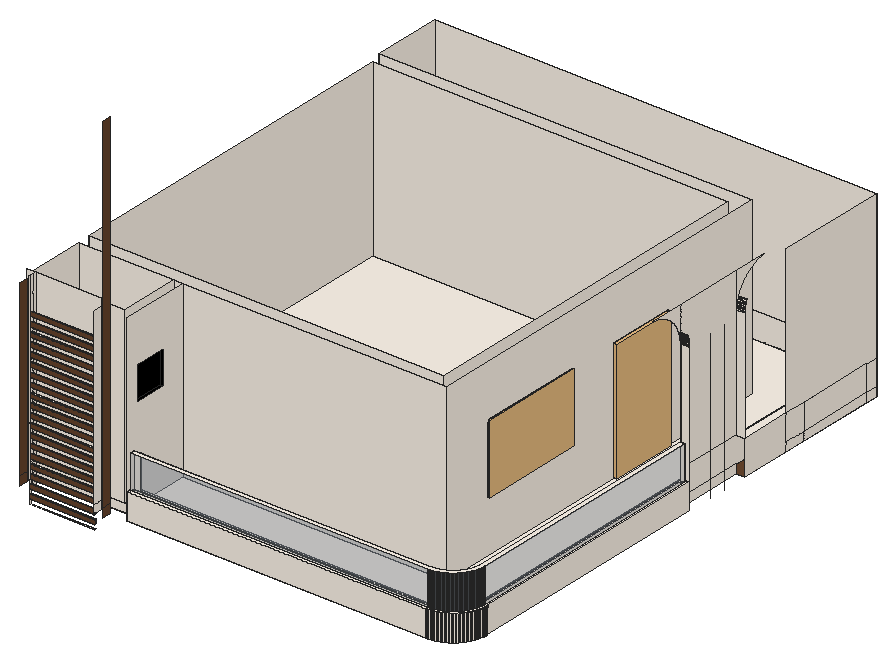
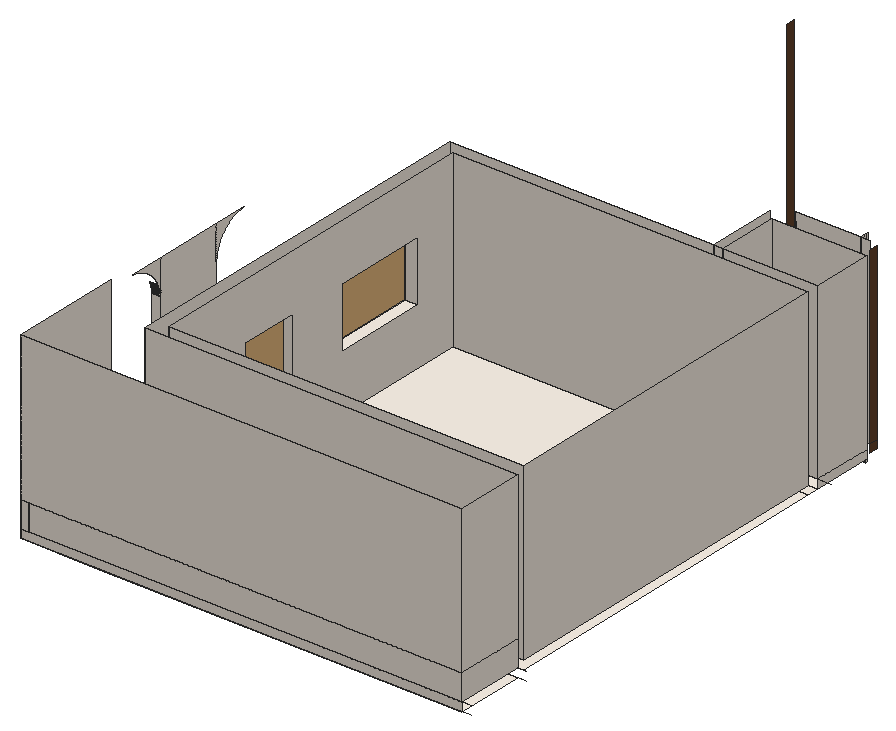
# SketchUp Ruby script. Lengths in inches.
U = 1.inch
M = Sketchup.active_model
def pt(a) = Geom::Point3d.new(a.map { |v| v * U })
def face(e, loops, mat)
  f = e.add_face(loops[0].map { |a| pt(a) })
  loops[1..].each { |l| e.add_face(l.map { |a| pt(a) }).erase! }
  f.material = f.back_material = mat if mat
  f
end
# faces: each face lists its corners as indices into pts; further lists are holes
def faces(e, pts, list, mat = nil) = list.each { |f| face(e, (f[0].is_a?(Array) ? f : [f]).map { |l| l.map { |i| pts[i] } }, mat) }
# xy, xz, yz: faces in a plane at the given z, y or x. An outline is a flat list of corners, or four numbers for a rectangle; further outlines are holes
def ring(l) = l.size == 4 ? [[l[0], l[1]], [l[2], l[1]], [l[2], l[3]], [l[0], l[3]]] : l.each_slice(2).to_a
def flat(e, list, mat, &to3) = list.each { |f| face(e, (f[0].is_a?(Array) ? f : [f]).map { |l| ring(l).map { |u, v| to3.(u, v) } }, mat) }
def xy(e, z, list, mat = nil) = flat(e, list, mat) { |x, y| [x, y, z] }
def xz(e, y, list, mat = nil) = flat(e, list, mat) { |x, z| [x, y, z] }
def yz(e, x, list, mat = nil) = flat(e, list, mat) { |y, z| [x, y, z] }
def lines(e, pts, list) = list.each { |a, b| e.add_line(pt(pts[a]), pt(pts[b])) }
# prism: a flat outline (further loops are holes) pulled along v
def prism(e, loops, v, mat = nil)
  f = face(e, loops, mat); d = Geom::Vector3d.new(v.map { |x| x * U })
  f.pushpull(f.normal.samedirection?(d) ? d.length : -d.length)
end
def box(e, o, s, mat = nil) = prism(e, [[o, [o[0] + s[0], o[1], o[2]], [o[0] + s[0], o[1] + s[1], o[2]], [o[0], o[1] + s[1], o[2]]]], [0, 0, s[2]], mat)
def at(x, y, z, deg = 0) = Geom::Transformation.translation(pt([x, y, z])) * Geom::Transformation.rotation(ORIGIN, Z_AXIS, deg.degrees)
def axes(o, x, y, z) = Geom::Transformation.new([*x, 0, *y, 0, *z, 0, *pt(o).to_a, 1])
def part(name) = M.definitions.add(name)
# library, detail: a bought-in or finely detailed component or shape, given as its bounding box
def library(name, o, s) = part(name).tap { |d| box(d.entities, o, s) }
def detail(e, o, s) = box(e.add_group.entities, o, s)
def put(e, d, t, mat = nil) = e.add_instance(d, t).tap { |i| i.material = mat if mat }
def group(e, t, mat = nil) = e.add_group.tap { |g| g.transformation = t; g.material = mat if mat }.entities
root = M.entities
M.materials.add("C01_Vanilla_Cream").color = [255, 246, 235]
M.materials.add("Glass_Basic_01").color = [161, 173, 186]
M.materials["Glass_Basic_01"].alpha = 0.25
M.materials.add("Wood_Veneer_15_1K").color = [103, 69, 45]
M.materials.add("[Color_009]1").color = [0, 0, 0]
c1 = library("porta+4",[0.2,-5.42,1.33],[46.55,4.72,83.21])
c2 = library("mesh-164",[-1582.71,-3144.16,-23.22],[2366.42,2227.34,65.81])
c3 = part("Group13")
put(c3.entities,c2,at(294.66,859.51,3.5))
xy(root,386.25,[[66,1,111,2]],"C01_Vanilla_Cream")
xy(root,389.4,[[66,1,111,2]],"C01_Vanilla_Cream")
xy(root,392.55,[[66,1,111,2]],"C01_Vanilla_Cream")
xy(root,395.7,[[66,1,111,2]],"C01_Vanilla_Cream")
xy(root,396,[[57,12,123,54],[123,12,129,54],[57,54,312,63],[57,63,303,309],[303,63,312,309],
  [54,318,312,366]],"C01_Vanilla_Cream")
xy(root,396,[[129,6,129,54,312,54,312,366,360,366,360,252,354,252,354,204,360,204,360,30,359.99,29.25,359.95,28.49,359.89,27.74,359.8125,26.99,359.7,26.25,359.57,25.5,359.42,24.76,359.25,24.03,359.05,23.3,358.83,22.58,358.58,21.87,358.31,21.17,358.03,20.47,357.72,19.78,357.38,19.1,357.03,18.4375,356.66,17.78,356.26,17.14,355.85,16.51,355.42,15.89,354.96,15.29,354.49,14.7,354,14.13,353.5,13.57,352.97,13.03,352.43,12.5,351.87,12,351.3,11.51,350.71,11.04,350.11,10.58,349.49,10.15,348.86,9.74,348.22,9.34,347.5625,8.97,346.9,8.62,346.22,8.28,345.53,7.97,344.83,7.69,344.13,7.42,343.42,7.17,342.7,6.95,341.97,6.75,341.24,6.58,340.5,6.43,339.75,6.3,339.01,6.1875,338.26,6.11,337.51,6.05,336.75,6.01,336,6]],"Wood_Veneer_15_1K")
xy(root,398.85,[[66,1,111,2]],"C01_Vanilla_Cream")
xy(root,402,[[66,1,111,2],[129,12,336,12,336.57,12.01,337.13,12.04,337.69,12.08,338.26,12.14,338.82,12.22,339.37,12.32,339.93,12.43,340.48,12.57,341.02,12.71,341.5625,12.88,342.1,13.0625,342.625,13.26,343.15,13.48,343.66,13.71,344.17,13.96,344.67,14.23,345.16,14.51,345.64,14.8,346.12,15.11,346.58,15.4375,347.03,15.78,347.47,16.13,347.9,16.5,348.32,16.88,348.73,17.27,349.12,17.68,349.5,18.1,349.87,18.53,350.22,18.97,350.5625,19.42,350.89,19.88,351.2,20.36,351.49,20.84,351.77,21.33,352.04,21.83,352.29,22.34,352.52,22.85,352.74,23.375,352.9375,23.9,353.12,24.4375,353.29,24.98,353.43,25.52,353.57,26.07,353.68,26.63,353.78,27.18,353.86,27.74,353.92,28.31,353.96,28.87,353.99,29.43,354,30,354,366,54,366,54,318,312,318,312,54,129,54],[57,12,123,54],[123,12,129,54],[57,63,303,309]],"C01_Vanilla_Cream")
xy(root,405,[[303,201,312,243]],"C01_Vanilla_Cream")
xy(root,405.15,[[66,1,111,2]],"C01_Vanilla_Cream")
xy(root,408.3,[[66,1,111,2]],"C01_Vanilla_Cream")
xy(root,411.45,[[66,1,111,2]],"C01_Vanilla_Cream")
xy(root,414,[[[129,6,336,6,336.75,6.01,337.51,6.05,338.26,6.11,339.01,6.1875,339.75,6.3,340.5,6.43,341.24,6.58,341.97,6.75,342.7,6.95,343.42,7.17,344.13,7.42,344.83,7.69,345.53,7.97,346.22,8.28,346.9,8.62,347.5625,8.97,348.22,9.34,348.86,9.74,349.49,10.15,350.11,10.58,350.71,11.04,351.3,11.51,351.87,12,352.43,12.5,352.97,13.03,353.5,13.57,354,14.13,354.49,14.7,354.96,15.29,355.42,15.89,355.85,16.51,356.26,17.14,356.66,17.78,357.03,18.4375,357.38,19.1,357.72,19.78,358.03,20.47,358.31,21.17,358.58,21.87,358.83,22.58,359.05,23.3,359.25,24.03,359.42,24.76,359.57,25.5,359.7,26.25,359.8125,26.99,359.89,27.74,359.95,28.49,359.99,29.25,360,30,360,204,354,204,354,30,353.99,29.43,353.96,28.87,353.92,28.31,353.86,27.74,353.78,27.18,353.68,26.63,353.57,26.07,353.43,25.52,353.29,24.98,353.12,24.4375,352.9375,23.9,352.74,23.375,352.52,22.85,352.29,22.34,352.04,21.83,351.77,21.33,351.49,20.84,351.2,20.36,350.89,19.88,350.5625,19.42,350.22,18.97,349.87,18.53,349.5,18.1,349.12,17.68,348.73,17.27,348.32,16.88,347.9,16.5,347.47,16.13,347.03,15.78,346.58,15.4375,346.12,15.11,345.64,14.8,345.16,14.51,344.67,14.23,344.17,13.96,343.66,13.71,343.15,13.48,342.625,13.26,342.1,13.0625,341.5625,12.88,341.02,12.71,340.48,12.57,339.93,12.43,339.37,12.32,338.82,12.22,338.26,12.14,337.69,12.08,337.13,12.04,336.57,12.01,336,12,129,12],[130.5,7.5,130.5,10.5,336,10.5,336.61,10.51,337.22,10.54,337.84,10.59,338.44,10.65,339.05,10.74,339.65,10.85,340.25,10.97,340.85,11.11,341.44,11.27,342.03,11.45,342.61,11.65,343.18,11.87,343.74,12.1,344.3,12.36,344.85,12.625,345.39,12.91,345.93,13.22,346.45,13.54,346.96,13.87,347.46,14.22,347.95,14.59,348.43,14.97,348.9,15.37,349.35,15.79,349.79,16.21,350.21,16.65,350.63,17.1,351.03,17.57,351.41,18.05,351.78,18.54,352.13,19.04,352.46,19.55,352.78,20.07,353.09,20.61,353.375,21.15,353.64,21.7,353.9,22.26,354.13,22.82,354.35,23.39,354.55,23.97,354.73,24.56,354.89,25.15,355.03,25.75,355.15,26.35,355.26,26.95,355.35,27.56,355.41,28.16,355.46,28.78,355.49,29.39,355.5,30,355.5,202.5,358.5,202.5,358.5,30,358.49,29.29,358.46,28.59,358.4,27.88,358.32,27.18,358.22,26.48,358.1,25.78,357.96,25.09,357.79,24.4,357.61,23.72,357.4,23.05,357.17,22.38,356.92,21.72,356.65,21.0625,356.36,20.42,356.05,19.79,355.72,19.16,355.37,18.55,355,17.94,354.61,17.35,354.2,16.77,353.78,16.21,353.34,15.66,352.88,15.12,352.4,14.6,351.91,14.09,351.4,13.6,350.88,13.12,350.34,12.66,349.79,12.22,349.23,11.8,348.65,11.39,348.06,11,347.45,10.63,346.84,10.28,346.21,9.95,345.58,9.64,344.9375,9.35,344.28,9.08,343.62,8.83,342.95,8.6,342.28,8.39,341.6,8.21,340.91,8.04,340.22,7.9,339.52,7.78,338.82,7.68,338.12,7.6,337.41,7.54,336.71,7.51,336,7.5]]],"C01_Vanilla_Cream")
xy(root,414.6,[[66,1,111,2]],"C01_Vanilla_Cream")
xy(root,417.75,[[66,1,111,2]],"C01_Vanilla_Cream")
xy(root,420,[[354,252,360,366]],"C01_Vanilla_Cream")
xy(root,420.9,[[66,1,111,2]],"C01_Vanilla_Cream")
xy(root,424.05,[[66,1,111,2]],"C01_Vanilla_Cream")
xy(root,427.2,[[66,1,111,2]],"C01_Vanilla_Cream")
xy(root,430.35,[[66,1,111,2]],"C01_Vanilla_Cream")
xy(root,433.5,[[66,1,111,2]],"C01_Vanilla_Cream")
xy(root,436.65,[[66,1,111,2]],"C01_Vanilla_Cream")
xy(root,438,[[130.5,7.5,336,7.5,336.71,7.51,337.41,7.54,338.12,7.6,338.82,7.68,339.52,7.78,340.22,7.9,340.91,8.04,341.6,8.21,342.28,8.39,342.95,8.6,343.62,8.83,344.28,9.08,344.9375,9.35,345.58,9.64,346.21,9.95,346.84,10.28,347.45,10.63,348.06,11,348.65,11.39,349.23,11.8,349.79,12.22,350.34,12.66,350.88,13.12,351.4,13.6,351.91,14.09,352.4,14.6,352.88,15.12,353.34,15.66,353.78,16.21,354.2,16.77,354.61,17.35,355,17.94,355.37,18.55,355.72,19.16,356.05,19.79,356.36,20.42,356.65,21.0625,356.92,21.72,357.17,22.38,357.4,23.05,357.61,23.72,357.79,24.4,357.96,25.09,358.1,25.78,358.22,26.48,358.32,27.18,358.4,27.88,358.46,28.59,358.49,29.29,358.5,30,358.5,202.5,355.5,202.5,355.5,30,355.49,29.39,355.46,28.78,355.41,28.16,355.35,27.56,355.26,26.95,355.15,26.35,355.03,25.75,354.89,25.15,354.73,24.56,354.55,23.97,354.35,23.39,354.13,22.82,353.9,22.26,353.64,21.7,353.375,21.15,353.09,20.61,352.78,20.07,352.46,19.55,352.13,19.04,351.78,18.54,351.41,18.05,351.03,17.57,350.63,17.1,350.21,16.65,349.79,16.21,349.35,15.79,348.9,15.37,348.43,14.97,347.95,14.59,347.46,14.22,346.96,13.87,346.45,13.54,345.93,13.22,345.39,12.91,344.85,12.625,344.3,12.36,343.74,12.1,343.18,11.87,342.61,11.65,342.03,11.45,341.44,11.27,340.85,11.11,340.25,10.97,339.65,10.85,339.05,10.74,338.44,10.65,337.84,10.59,337.22,10.54,336.61,10.51,336,10.5,130.5,10.5]],"C01_Vanilla_Cream")
xy(root,439.8,[[66,1,111,2]],"C01_Vanilla_Cream")
xy(root,441,[[303,93,312,159]],"C01_Vanilla_Cream")
xy(root,442.95,[[66,1,111,2]],"C01_Vanilla_Cream")
xy(root,446.1,[[66,1,111,2]],"C01_Vanilla_Cream")
xy(root,449.25,[[66,1,111,2]],"C01_Vanilla_Cream")
xy(root,452.4,[[66,1,111,2]],"C01_Vanilla_Cream")
xy(root,455.55,[[66,1,111,2]],"C01_Vanilla_Cream")
xy(root,458.7,[[66,1,111,2]],"C01_Vanilla_Cream")
xy(root,461.85,[[66,1,111,2]],"C01_Vanilla_Cream")
xy(root,465,[[66,1,111,2]],"C01_Vanilla_Cream")
xy(root,465.19,[[126,14.34,129,38.34]],"[Color_009]1")
xy(root,468.15,[[66,1,111,2]],"C01_Vanilla_Cream")
xy(root,471.3,[[66,1,111,2]],"C01_Vanilla_Cream")
xy(root,474.45,[[66,1,111,2]],"C01_Vanilla_Cream")
xy(root,477.6,[[66,1,111,2]],"C01_Vanilla_Cream")
xy(root,480.75,[[66,1,111,2]],"C01_Vanilla_Cream")
xy(root,483,[[303,93,312,159],[303,201,312,243]],"C01_Vanilla_Cream")
xy(root,483.9,[[66,1,111,2]],"C01_Vanilla_Cream")
xy(root,487.05,[[66,1,111,2]],"C01_Vanilla_Cream")
xy(root,489.19,[[126,14.34,129,38.34]],"[Color_009]1")
xy(root,490.2,[[66,1,111,2]],"C01_Vanilla_Cream")
xy(root,493.35,[[66,1,111,2]],"C01_Vanilla_Cream")
xy(root,496.5,[[66,1,111,2]],"C01_Vanilla_Cream")
xy(root,499.65,[[66,1,111,2]],"C01_Vanilla_Cream")
xy(root,502.8,[[66,1,111,2]],"C01_Vanilla_Cream")
xz(root,1,[[66,389.4,111,392.55],[66,395.7,111,398.85],[66,402,111,405.15],[66,408.3,111,411.45],[66,414.6,111,417.75],
  [66,420.9,111,424.05],[66,427.2,111,430.35],[66,433.5,111,436.65],[66,439.8,111,442.95],[66,446.1,111,449.25],
  [66,452.4,111,455.55],[66,458.7,111,461.85],[66,465,111,468.15],[66,471.3,111,474.45],[66,477.6,111,480.75],
  [66,483.9,111,487.05],[66,490.2,111,493.35],[66,496.5,111,499.65],[66,502.8,111,505.95]],"Wood_Veneer_15_1K")
xz(root,2,[[66,389.4,111,392.55],[66,395.7,111,396],[66,396,111,398.85],[66,402,111,405.15],[66,408.3,111,411.45],
  [66,414.6,111,417.75],[66,420.9,111,424.05],[66,427.2,111,430.35],[66,433.5,111,436.65],[66,439.8,111,442.95],
  [66,446.1,111,449.25],[66,452.4,111,455.55],[66,458.7,111,461.85],[66,465,111,468.15],[66,471.3,111,474.45],
  [66,477.6,111,480.75],[66,483.9,111,487.05],[66,490.2,111,493.35],[66,496.5,111,499.65],[66,502.8,111,505.95]],"C01_Vanilla_Cream")
xz(root,6,[[129,396,336,414],[60,402,66,528],[66,402,111,528]],"C01_Vanilla_Cream")
xz(root,7.5,[[130.5,414,336,438]],"Glass_Basic_01")
xz(root,10.5,[[130.5,414,135,438]],"C01_Vanilla_Cream")
xz(root,10.5,[[135,414,336,438]],"Glass_Basic_01")
xz(root,12,[[57,396,129,402],[57,402,123,522],[129,402,135,414],[135,402,336,414]],"C01_Vanilla_Cream")
xz(root,14.34,[[126,465.19,129,489.19]],"[Color_009]1")
xz(root,38.34,[[126,465.19,129,489.19]],"[Color_009]1")
xz(root,54,[[57,402,123,522],[123,402,129,522],[129,402,312,522]],"C01_Vanilla_Cream")
xz(root,63,[[57,402,303,522]],"C01_Vanilla_Cream")
xz(root,93,[[303,441,312,483]],"C01_Vanilla_Cream")
xz(root,159,[[303,441,312,483]],"C01_Vanilla_Cream")
xz(root,201,[[303,405,312,483]],"C01_Vanilla_Cream")
xz(root,202.5,[[355.5,414,358.5,438]],"C01_Vanilla_Cream")
xz(root,204,[[354,396,360,414],[354,414,360,498]],"C01_Vanilla_Cream")
xz(root,243,[[303,405,312,483]],"C01_Vanilla_Cream")
xz(root,252,[[354,420,360,498]],"C01_Vanilla_Cream")
xz(root,309,[[57,402,303,522]],"C01_Vanilla_Cream")
xz(root,318,[[54,402,312,522]],"C01_Vanilla_Cream")
xz(root,366,[[54,396,360,402],[54,402,354,420],[354,402,360,420],[54,420,360,522]],"C01_Vanilla_Cream")
yz(root,54,[[318,402,366,420],[318,420,366,522]],"C01_Vanilla_Cream")
yz(root,57,[[12,396,54,402],[12,402,54,522],[63,402,309,522]],"C01_Vanilla_Cream")
yz(root,60,[[0,396,6,402],[0,402,6,522]],"Wood_Veneer_15_1K")
yz(root,66,[[1,386.25,2,389.4],[1,392.55,2,395.7],[3,396,6,402],[1,398.85,2,402],[0,402,1,528],
  [2,402,3,528],[3,402,6,528],[1,405.15,2,408.3],[1,411.45,2,414.6],[1,417.75,2,420.9],
  [1,424.05,2,427.2],[1,430.35,2,433.5],[1,436.65,2,439.8],[1,442.95,2,446.1],[1,449.25,2,452.4],
  [1,455.55,2,458.7],[1,461.85,2,465],[1,468.15,2,471.3],[1,474.45,2,477.6],[1,480.75,2,483.9],
  [1,487.05,2,490.2],[1,493.35,2,496.5],[1,499.65,2,502.8]],"C01_Vanilla_Cream")
yz(root,111,[[1,395.7,2,396],[0,396,0,402,6,402,6,396,2,396,2,398.85,1,398.85,1,396],[1,396,2,398.85],[[0,402,0,522,1,522,1,521.7,2,521.7,2,522,6,522,6,402,2,402,2,405.15,1,405.15,1,402],[1,490.2,2,493.35],[1,483.9,2,487.05],[1,465,2,468.15],[1,458.7,2,461.85],[1,452.4,2,455.55],[1,446.1,2,449.25],[1,439.8,2,442.95],[1,433.5,2,436.65],[1,427.2,2,430.35],[1,420.9,2,424.05],[1,414.6,2,417.75],[1,408.3,2,411.45],[1,515.4,2,518.55],[1,509.1,2,512.25],[1,502.8,2,505.95],[1,496.5,2,499.65],[1,477.6,2,480.75],[1,471.3,2,474.45]]],"C01_Vanilla_Cream")
yz(root,117,[[0,396,6,402],[0,402,6,642]],"Wood_Veneer_15_1K")
yz(root,123,[[12,402,54,522]],"C01_Vanilla_Cream")
yz(root,126,[[14.34,465.19,38.34,489.19]],"[Color_009]1")
yz(root,129,[[6,396,12,402],[6,402,12,414],[[12,402,54,402,54,522,6,522,6,414,12,414],[14.34,465.19,38.34,489.19]]],"C01_Vanilla_Cream")
yz(root,130.5,[[7.5,414,10.5,438]],"C01_Vanilla_Cream")
yz(root,303,[[[63,402,309,522],[201,405,243,483],[93,441,159,483]]],"C01_Vanilla_Cream")
yz(root,312,[[[54,402,198,402,198,486,246,486,246,402,318,402,318,522,54,522],[90,438,162,486]],[[198,402,246,486],[201,405,243,483]],[[90,438,162,486],[93,441,159,483]]],"C01_Vanilla_Cream")
yz(root,354,[[204,396,252,402],[30,402,204,414],[204,402,366,420],[204,420,252,522],[204,498,203.96,498.75,203.9,499.49,203.82,500.23,203.71,500.97,203.58,501.71,203.44,502.4375,203.26,503.16,203.07,503.89,202.86,504.6,202.62,505.31,202.36,506.01,202.09,506.7,201.79,507.39,201.47,508.0625,201.13,508.73,200.77,509.38,200.39,510.03,200,510.66,199.58,511.28,199.15,511.89,198.69,512.48,198.22,513.0625,197.74,513.625,197.23,514.18,196.71,514.71,196.18,515.23,195.625,515.74,195.0625,516.22,194.48,516.69,193.89,517.15,193.28,517.58,192.66,518,192.03,518.39,191.38,518.77,190.73,519.13,190.0625,519.47,189.39,519.79,188.7,520.09,188.01,520.36,187.31,520.62,186.6,520.86,185.89,521.07,185.16,521.26,184.4375,521.44,183.71,521.58,182.97,521.71,182.23,521.82,181.49,521.9,180.75,521.96,180,522,204,522],
  [252,498,252,522,276,522,275.27,521.92,274.54,521.82,273.8125,521.71,273.09,521.57,272.37,521.41,271.65,521.23,270.94,521.03,270.24,520.82,269.54,520.58,268.85,520.32,268.17,520.05,267.5,519.75,266.83,519.44,266.17,519.11,265.52,518.76,264.88,518.39,264.26,518.01,263.64,517.61,263.03,517.1875,262.44,516.75,261.86,516.3,261.29,515.83,260.73,515.35,260.19,514.85,259.66,514.34,259.15,513.81,258.65,513.27,258.17,512.71,257.7,512.14,257.25,511.56,256.8125,510.97,256.39,510.36,255.99,509.74,255.61,509.12,255.24,508.48,254.89,507.83,254.56,507.17,254.25,506.5,253.95,505.83,253.68,505.15,253.42,504.46,253.18,503.76,252.97,503.06,252.77,502.35,252.59,501.63,252.43,500.91,252.29,500.1875,252.18,499.46,252.08,498.73]],"C01_Vanilla_Cream")
yz(root,355.5,[[30,414,202.5,438]],"Glass_Basic_01")
yz(root,358.5,[[30,414,202.5,438]],"Glass_Basic_01")
yz(root,360,[[30,396,204,414],[252,396,288,420],[288,396,303,402],[303,396,357,402],[357,396,366,402],
  [288,402,303,420],[303,402,357,420],[357,402,366,420],[288,420,366,522]],"C01_Vanilla_Cream")
p = [[336.75,6.01,396],[336.75,6.01,414],[336,6,414],[336,6,396],[337.51,6.05,396],[337.51,6.05,414],
  [338.26,6.11,396],[338.26,6.11,414],[339.01,6.1875,396],[339.01,6.1875,414],[339.75,6.3,396],[339.75,6.3,414],
  [340.5,6.43,396],[340.5,6.43,414],[341.24,6.58,396],[341.24,6.58,414],[341.97,6.75,396],[341.97,6.75,414],
  [342.7,6.95,396],[342.7,6.95,414],[343.42,7.17,396],[343.42,7.17,414],[344.13,7.42,396],[344.13,7.42,414],
  [344.83,7.69,396],[344.83,7.69,414],[345.53,7.97,396],[345.53,7.97,414],[346.22,8.28,396],[346.22,8.28,414],
  [346.9,8.62,396],[346.9,8.62,414],[347.5625,8.97,396],[347.5625,8.97,414],[348.22,9.34,396],[348.22,9.34,414],
  [348.86,9.74,396],[348.86,9.74,414],[349.49,10.15,396],[349.49,10.15,414],[350.11,10.58,396],[350.11,10.58,414],
  [350.71,11.04,396],[350.71,11.04,414],[351.3,11.51,396],[351.3,11.51,414],[351.87,12,396],[351.87,12,414],
  [352.43,12.5,396],[352.43,12.5,414],[352.97,13.03,396],[352.97,13.03,414],[353.5,13.57,396],[353.5,13.57,414],
  [354,14.13,396],[354,14.13,414],[354.49,14.7,396],[354.49,14.7,414],[354.96,15.29,396],[354.96,15.29,414],
  [355.42,15.89,396],[355.42,15.89,414],[355.85,16.51,396],[355.85,16.51,414],[356.26,17.14,396],[356.26,17.14,414],
  [356.66,17.78,396],[356.66,17.78,414],[357.03,18.4375,396],[357.03,18.4375,414],[357.38,19.1,396],[357.38,19.1,414],
  [357.72,19.78,396],[357.72,19.78,414],[358.03,20.47,396],[358.03,20.47,414],[358.31,21.17,396],[358.31,21.17,414],
  [358.58,21.87,396],[358.58,21.87,414],[358.83,22.58,396],[358.83,22.58,414],[359.05,23.3,396],[359.05,23.3,414],
  [359.25,24.03,396],[359.25,24.03,414],[359.42,24.76,396],[359.42,24.76,414],[359.57,25.5,396],[359.57,25.5,414],
  [359.7,26.25,396],[359.7,26.25,414],[359.8125,26.99,396],[359.8125,26.99,414],[359.89,27.74,396],[359.89,27.74,414],
  [359.95,28.49,396],[359.95,28.49,414],[359.99,29.25,396],[359.99,29.25,414],[360,30,396],[360,30,414],
  [336.57,12.01,402],[336,12,402],[336,12,414],[336.57,12.01,414],[337.13,12.04,402],[337.13,12.04,414],
  [337.69,12.08,402],[337.69,12.08,414],[338.26,12.14,402],[338.26,12.14,414],[338.82,12.22,402],[338.82,12.22,414],
  [339.37,12.32,402],[339.37,12.32,414],[339.93,12.43,402],[339.93,12.43,414],[340.48,12.57,402],[340.48,12.57,414],
  [341.02,12.71,402],[341.02,12.71,414],[341.5625,12.88,402],[341.5625,12.88,414],[342.1,13.0625,402],[342.1,13.0625,414],
  [342.625,13.26,402],[342.625,13.26,414],[343.15,13.48,402],[343.15,13.48,414],[343.66,13.71,402],[343.66,13.71,414],
  [344.17,13.96,402],[344.17,13.96,414],[344.67,14.23,402],[344.67,14.23,414],[345.16,14.51,402],[345.16,14.51,414],
  [345.64,14.8,402],[345.64,14.8,414],[346.12,15.11,402],[346.12,15.11,414],[346.58,15.4375,402],[346.58,15.4375,414],
  [347.03,15.78,402],[347.03,15.78,414],[347.47,16.13,402],[347.47,16.13,414],[347.9,16.5,402],[347.9,16.5,414],
  [348.32,16.88,402],[348.32,16.88,414],[348.73,17.27,402],[348.73,17.27,414],[349.12,17.68,402],[349.12,17.68,414],
  [349.5,18.1,402],[349.5,18.1,414],[349.87,18.53,402],[349.87,18.53,414],[350.22,18.97,402],[350.22,18.97,414],
  [350.5625,19.42,402],[350.5625,19.42,414],[350.89,19.88,402],[350.89,19.88,414],[351.2,20.36,402],[351.2,20.36,414],
  [351.49,20.84,402],[351.49,20.84,414],[351.77,21.33,402],[351.77,21.33,414],[352.04,21.83,402],[352.04,21.83,414],
  [352.29,22.34,402],[352.29,22.34,414],[352.52,22.85,402],[352.52,22.85,414],[352.74,23.375,402],[352.74,23.375,414],
  [352.9375,23.9,402],[352.9375,23.9,414],[353.12,24.4375,402],[353.12,24.4375,414],[353.29,24.98,402],[353.29,24.98,414],
  [353.43,25.52,402],[353.43,25.52,414],[353.57,26.07,402],[353.57,26.07,414],[353.68,26.63,402],[353.68,26.63,414],
  [353.78,27.18,402],[353.78,27.18,414],[353.86,27.74,402],[353.86,27.74,414],[353.92,28.31,402],[353.92,28.31,414],
  [353.96,28.87,402],[353.96,28.87,414],[353.99,29.43,402],[353.99,29.43,414],[354,30,402],[354,30,414],
  [336,7.5,414],[336.71,7.51,414],[336.71,7.51,438],[336,7.5,438],[337.41,7.54,414],[337.41,7.54,438],
  [338.12,7.6,414],[338.12,7.6,438],[338.82,7.68,414],[338.82,7.68,438],[339.52,7.78,414],[339.52,7.78,438],
  [340.22,7.9,414],[340.22,7.9,438],[340.91,8.04,414],[340.91,8.04,438],[341.6,8.21,414],[341.6,8.21,438],
  [342.28,8.39,414],[342.28,8.39,438],[342.95,8.6,414],[342.95,8.6,438],[343.62,8.83,414],[343.62,8.83,438],
  [344.28,9.08,414],[344.28,9.08,438],[344.9375,9.35,414],[344.9375,9.35,438],[345.58,9.64,414],[345.58,9.64,438],
  [346.21,9.95,414],[346.21,9.95,438],[346.84,10.28,414],[346.84,10.28,438],[347.45,10.63,414],[347.45,10.63,438],
  [336.61,10.51,414],[336,10.5,414],[336,10.5,438],[336.61,10.51,438],[337.22,10.54,414],[337.22,10.54,438],
  [337.84,10.59,414],[337.84,10.59,438],[338.44,10.65,414],[338.44,10.65,438],[348.06,11,414],[348.06,11,438],
  [339.05,10.74,414],[339.05,10.74,438],[339.65,10.85,414],[339.65,10.85,438],[340.25,10.97,414],[340.25,10.97,438],
  [340.85,11.11,414],[340.85,11.11,438],[348.65,11.39,414],[348.65,11.39,438],[341.44,11.27,414],[341.44,11.27,438],
  [342.03,11.45,414],[342.03,11.45,438],[349.23,11.8,414],[349.23,11.8,438],[342.61,11.65,414],[342.61,11.65,438],
  [343.18,11.87,414],[343.18,11.87,438],[349.79,12.22,414],[349.79,12.22,438],[343.74,12.1,414],[343.74,12.1,438],
  [344.3,12.36,414],[344.3,12.36,438],[350.34,12.66,414],[350.34,12.66,438],[344.85,12.625,414],[344.85,12.625,438],
  [345.39,12.91,414],[345.39,12.91,438],[350.88,13.12,414],[350.88,13.12,438],[345.93,13.22,414],[345.93,13.22,438],
  [351.4,13.6,414],[351.4,13.6,438],[346.45,13.54,414],[346.45,13.54,438],[346.96,13.87,414],[346.96,13.87,438],
  [351.91,14.09,414],[351.91,14.09,438],[347.46,14.22,414],[347.46,14.22,438],[352.4,14.6,414],[352.4,14.6,438],
  [347.95,14.59,414],[347.95,14.59,438],[348.43,14.97,414],[348.43,14.97,438],[352.88,15.12,414],[352.88,15.12,438],
  [348.9,15.37,414],[348.9,15.37,438],[353.34,15.66,414],[353.34,15.66,438],[349.35,15.79,414],[349.35,15.79,438],
  [353.78,16.21,414],[353.78,16.21,438],[349.79,16.21,414],[349.79,16.21,438],[350.21,16.65,414],[350.21,16.65,438],
  [354.2,16.77,414],[354.2,16.77,438],[350.63,17.1,414],[350.63,17.1,438],[354.61,17.35,414],[354.61,17.35,438],
  [351.03,17.57,414],[351.03,17.57,438],[355,17.94,414],[355,17.94,438],[351.41,18.05,414],[351.41,18.05,438],
  [355.37,18.55,414],[355.37,18.55,438],[351.78,18.54,414],[351.78,18.54,438],[352.13,19.04,414],[352.13,19.04,438],
  [355.72,19.16,414],[355.72,19.16,438],[352.46,19.55,414],[352.46,19.55,438],[356.05,19.79,414],[356.05,19.79,438],
  [352.78,20.07,414],[352.78,20.07,438],[356.36,20.42,414],[356.36,20.42,438],[353.09,20.61,414],[353.09,20.61,438],
  [356.65,21.0625,414],[356.65,21.0625,438],[353.375,21.15,414],[353.375,21.15,438],[353.64,21.7,414],[353.64,21.7,438],
  [356.92,21.72,414],[356.92,21.72,438],[353.9,22.26,414],[353.9,22.26,438],[357.17,22.38,414],[357.17,22.38,438],
  [354.13,22.82,414],[354.13,22.82,438],[357.4,23.05,414],[357.4,23.05,438],[354.35,23.39,414],[354.35,23.39,438],
  [357.61,23.72,414],[357.61,23.72,438],[354.55,23.97,414],[354.55,23.97,438],[357.79,24.4,414],[357.79,24.4,438],
  [354.73,24.56,414],[354.73,24.56,438],[357.96,25.09,414],[357.96,25.09,438],[354.89,25.15,414],[354.89,25.15,438],
  [358.1,25.78,414],[358.1,25.78,438],[355.03,25.75,414],[355.03,25.75,438],[355.15,26.35,414],[355.15,26.35,438],
  [358.22,26.48,414],[358.22,26.48,438],[355.26,26.95,414],[355.26,26.95,438],[358.32,27.18,414],[358.32,27.18,438],
  [355.35,27.56,414],[355.35,27.56,438],[358.4,27.88,414],[358.4,27.88,438],[355.41,28.16,414],[355.41,28.16,438],
  [358.46,28.59,414],[358.46,28.59,438],[355.46,28.78,414],[355.46,28.78,438],[358.49,29.29,414],[358.49,29.29,438],
  [355.49,29.39,414],[355.49,29.39,438],[358.5,30,414],[358.5,30,438],[355.5,30,414],[355.5,30,438],
  [360,204,498],[360,203.96,498.75],[354,203.96,498.75],[354,204,498],[360,252.08,498.73],[360,252,498],
  [354,252,498],[354,252.08,498.73],[360,203.9,499.49],[354,203.9,499.49],[360,252.18,499.46],[354,252.18,499.46],
  [360,203.82,500.23],[354,203.82,500.23],[360,252.29,500.1875],[354,252.29,500.1875],[360,203.71,500.97],[354,203.71,500.97],
  [360,252.43,500.91],[354,252.43,500.91],[360,252.59,501.63],[354,252.59,501.63],[360,203.58,501.71],[354,203.58,501.71],
  [360,252.77,502.35],[354,252.77,502.35],[360,203.44,502.4375],[354,203.44,502.4375],[360,252.97,503.06],[354,252.97,503.06],
  [360,203.26,503.16],[354,203.26,503.16],[360,253.18,503.76],[354,253.18,503.76],[360,203.07,503.89],[354,203.07,503.89],
  [360,253.42,504.46],[354,253.42,504.46],[360,202.86,504.6],[354,202.86,504.6],[360,253.68,505.15],[354,253.68,505.15],
  [360,202.62,505.31],[354,202.62,505.31],[360,253.95,505.83],[354,253.95,505.83],[360,202.36,506.01],[354,202.36,506.01],
  [48,318,396],[54,318,396],[48,318,402],[54,318,402],[57,54,402],[48,54,402],
  [360,222,414],[360,222,396],[360,221.99,498.33],[360,234,396],[360,234,420],[360,234,498.48],
  [54,366,402],[48,366,402],[54,366,396],[48,366,396]]
faces(root,p,[[0,1,2,3],[4,5,1,0],[6,7,5,4],[8,9,7,6],[10,11,9,8],[12,13,11,10],[14,15,13,12],[16,17,15,14],
  [18,19,17,16],[20,21,19,18],[22,23,21,20],[24,25,23,22],[26,27,25,24],[28,29,27,26],[30,31,29,28],[32,33,31,30],
  [34,35,33,32],[36,37,35,34],[38,39,37,36],[40,41,39,38],[42,43,41,40],[44,45,43,42],[46,47,45,44],[48,49,47,46],
  [50,51,49,48],[52,53,51,50],[54,55,53,52],[56,57,55,54],[58,59,57,56],[60,61,59,58],[62,63,61,60],[64,65,63,62],
  [66,67,65,64],[68,69,67,66],[70,71,69,68],[72,73,71,70],[74,75,73,72],[76,77,75,74],[78,79,77,76],[80,81,79,78],
  [82,83,81,80],[84,85,83,82],[86,87,85,84],[88,89,87,86],[90,91,89,88],[92,93,91,90],[94,95,93,92],[96,97,95,94],
  [98,99,97,96],[100,101,99,98],[102,103,104,105],[106,102,105,107],[108,106,107,109],[110,108,109,111],[112,110,111,113],[114,112,113,115],
  [116,114,115,117],[118,116,117,119],[120,118,119,121],[122,120,121,123],[124,122,123,125],[126,124,125,127],[128,126,127,129],[130,128,129,131],
  [132,130,131,133],[134,132,133,135],[136,134,135,137],[138,136,137,139],[140,138,139,141],[142,140,141,143],[144,142,143,145],[146,144,145,147],
  [148,146,147,149],[150,148,149,151],[152,150,151,153],[154,152,153,155],[156,154,155,157],[158,156,157,159],[160,158,159,161],[162,160,161,163],
  [164,162,163,165],[166,164,165,167],[168,166,167,169],[170,168,169,171],[172,170,171,173],[174,172,173,175],[176,174,175,177],[178,176,177,179],
  [180,178,179,181],[182,180,181,183],[184,182,183,185],[186,184,185,187],[188,186,187,189],[190,188,189,191],[192,190,191,193],[194,192,193,195],
  [196,194,195,197],[198,196,197,199],[200,198,199,201],[202,200,201,203],[408,409,410,411],[412,413,414,415],[409,416,417,410],[418,412,415,419],
  [416,420,421,417],[422,418,419,423],[420,424,425,421],[426,422,423,427],[428,426,427,429],[424,430,431,425],[432,428,429,433],[430,434,435,431],
  [436,432,433,437],[434,438,439,435],[440,436,437,441],[438,442,443,439],[444,440,441,445],[442,446,447,443],[448,444,445,449],[446,450,451,447],
  [452,448,449,453],[450,454,455,451]],"C01_Vanilla_Cream")
faces(root,p,[[204,205,206,207],[205,208,209,206],[208,210,211,209],[210,212,213,211],[212,214,215,213],[214,216,217,215],[216,218,219,217],[218,220,221,219],
  [220,222,223,221],[222,224,225,223],[224,226,227,225],[226,228,229,227],[228,230,231,229],[230,232,233,231],[232,234,235,233],[234,236,237,235],
  [236,238,239,237],[240,241,242,243],[244,240,243,245],[246,244,245,247],[248,246,247,249],[238,250,251,239],[252,248,249,253],[254,252,253,255],
  [256,254,255,257],[258,256,257,259],[250,260,261,251],[262,258,259,263],[264,262,263,265],[260,266,267,261],[268,264,265,269],[270,268,269,271],
  [266,272,273,267],[274,270,271,275],[276,274,275,277],[272,278,279,273],[280,276,277,281],[282,280,281,283],[278,284,285,279],[286,282,283,287],
  [284,288,289,285],[290,286,287,291],[292,290,291,293],[288,294,295,289],[296,292,293,297],[294,298,299,295],[300,296,297,301],[302,300,301,303],
  [298,304,305,299],[306,302,303,307],[304,308,309,305],[310,306,307,311],[308,312,313,309],[314,310,311,315],[316,314,315,317],[312,318,319,313],
  [320,316,317,321],[318,322,323,319],[324,320,321,325],[322,326,327,323],[328,324,325,329],[326,330,331,327],[332,328,329,333],[334,332,333,335],
  [330,336,337,331],[338,334,335,339],[336,340,341,337],[342,338,339,343],[340,344,345,341],[346,342,343,347],[344,348,349,345],[350,346,347,351],
  [352,350,351,353],[348,354,355,349],[356,352,353,357],[354,358,359,355],[360,356,357,361],[358,362,363,359],[364,360,361,365],[362,366,367,363],
  [368,364,365,369],[366,370,371,367],[372,368,369,373],[370,374,375,371],[376,372,373,377],[374,378,379,375],[380,376,377,381],[382,380,381,383],
  [378,384,385,379],[386,382,383,387],[384,388,389,385],[390,386,387,391],[388,392,393,389],[394,390,391,395],[392,396,397,393],[398,394,395,399],
  [396,400,401,397],[402,398,399,403],[400,404,405,401],[406,402,403,407]],"Glass_Basic_01")
lines(root,p,[[456,457],[458,459],[460,461],[462,463],[464,462],[465,466],[466,467],[468,469],[470,471]])
put(root,c1,at(309.24,197.8,401.48,90))
put(root,c3,axes([312.39,129.3,487.23],[0,0.03051,0],[0,0,0.02146],[0.01969,0,0]))
